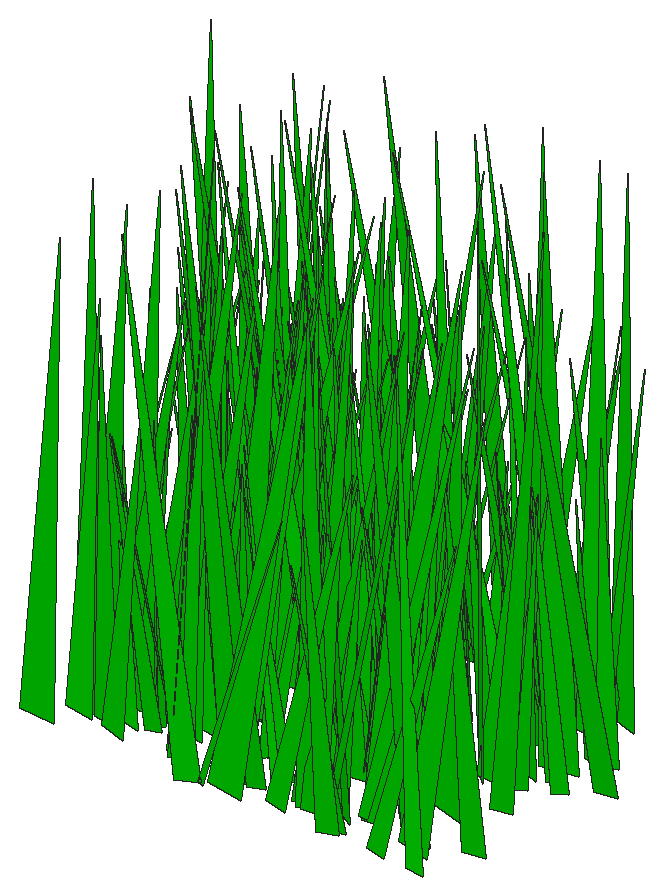
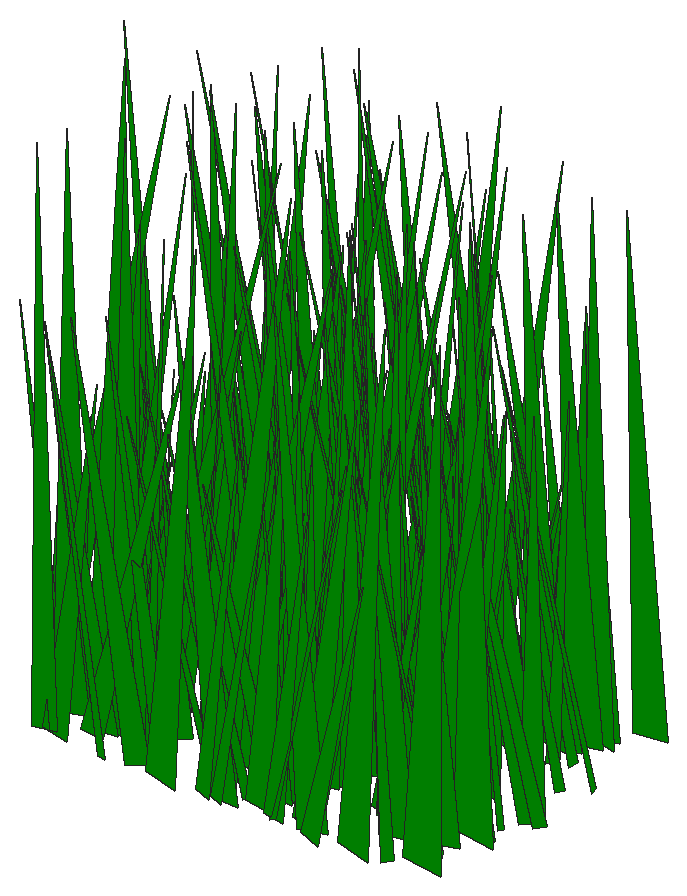
# SketchUp Ruby script. Lengths in inches.
U = 1.inch
M = Sketchup.active_model
def pt(a) = Geom::Point3d.new(a.map { |v| v * U })
def face(e, loops, mat)
  f = e.add_face(loops[0].map { |a| pt(a) })
  loops[1..].each { |l| e.add_face(l.map { |a| pt(a) }).erase! }
  f.material = f.back_material = mat if mat
  f
end
# faces: each face lists its corners as indices into pts; further lists are holes
def faces(e, pts, list, mat = nil) = list.each { |f| face(e, (f[0].is_a?(Array) ? f : [f]).map { |l| l.map { |i| pts[i] } }, mat) }
# xy, xz, yz: faces in a plane at the given z, y or x. An outline is a flat list of corners, or four numbers for a rectangle; further outlines are holes
def ring(l) = l.size == 4 ? [[l[0], l[1]], [l[2], l[1]], [l[2], l[3]], [l[0], l[3]]] : l.each_slice(2).to_a
def flat(e, list, mat, &to3) = list.each { |f| face(e, (f[0].is_a?(Array) ? f : [f]).map { |l| ring(l).map { |u, v| to3.(u, v) } }, mat) }
def xy(e, z, list, mat = nil) = flat(e, list, mat) { |x, y| [x, y, z] }
def xz(e, y, list, mat = nil) = flat(e, list, mat) { |x, z| [x, y, z] }
def yz(e, x, list, mat = nil) = flat(e, list, mat) { |y, z| [x, y, z] }
def lines(e, pts, list) = list.each { |a, b| e.add_line(pt(pts[a]), pt(pts[b])) }
# prism: a flat outline (further loops are holes) pulled along v
def prism(e, loops, v, mat = nil)
  f = face(e, loops, mat); d = Geom::Vector3d.new(v.map { |x| x * U })
  f.pushpull(f.normal.samedirection?(d) ? d.length : -d.length)
end
def box(e, o, s, mat = nil) = prism(e, [[o, [o[0] + s[0], o[1], o[2]], [o[0] + s[0], o[1] + s[1], o[2]], [o[0], o[1] + s[1], o[2]]]], [0, 0, s[2]], mat)
def at(x, y, z, deg = 0) = Geom::Transformation.translation(pt([x, y, z])) * Geom::Transformation.rotation(ORIGIN, Z_AXIS, deg.degrees)
def axes(o, x, y, z) = Geom::Transformation.new([*x, 0, *y, 0, *z, 0, *pt(o).to_a, 1])
def part(name) = M.definitions.add(name)
# library, detail: a bought-in or finely detailed component or shape, given as its bounding box
def library(name, o, s) = part(name).tap { |d| box(d.entities, o, s) }
def detail(e, o, s) = box(e.add_group.entities, o, s)
def put(e, d, t, mat = nil) = e.add_instance(d, t).tap { |i| i.material = mat if mat }
def group(e, t, mat = nil) = e.add_group.tap { |g| g.transformation = t; g.material = mat if mat }.entities
root = M.entities
M.materials.add("[Color G06]").color = [0, 204, 0]
c1 = part("fur_instance\#9")
p = [[0.8125,0,1.79],[0.67,-0.02,1.48],[0,-0.11,0],[0,0.11,0]]
faces(c1.entities,p,[[0,1,2,3]])
put(root,c1,axes([79.69,23.12,4.28],[1.66011,0.80063,2.32778],[5.89187,-0.25245,0.58844],[-0.82253,-0.19243,8.91321]),"[Color G06]")
put(root,c1,axes([79.5,20.96,4.28],[1.87537,-0.4948,0.57966],[-3.50181,-0.26688,-0.86236],[-0.69185,0.00955,5.93611]),"[Color G06]")
put(root,c1,axes([79.8125,25.06,4.28],[0.92833,-0.7609,0.17806],[-5.43768,-0.13039,-0.6811],[-0.46928,0.00566,8.24438]),"[Color G06]")
put(root,c1,axes([80.91,22.99,4.28],[-1.65961,0.74397,0.46911],[5.32789,0.22671,0.80106],[-0.4198,-0.06384,8.31219]),"[Color G06]")
put(root,c1,axes([79.46,16.25,4.28],[0.84063,-0.68793,1.84185],[-5.08275,-0.10859,0.52278],[0.14861,0.17743,7.46121]),"[Color G06]")
put(root,c1,axes([79.29,22.84,4.28],[3.77502,-0.05188,0.90133],[-0.29369,-0.5294,-0.7527],[-0.64486,-0.06259,5.61919]),"[Color G06]")
put(root,c1,axes([79.43,22.34,4.28],[4.54838,0.15375,1.99844],[1.30213,-0.64875,-0.88622],[-1.14373,-0.12715,6.93841]),"[Color G06]")
put(root,c1,axes([80.61,18.76,4.28],[-3.18523,0.26777,1.23981],[1.8153,0.45856,-0.9593],[1.0393,0.01971,5.47532]),"[Color G06]")
put(root,c1,axes([79.5,19.875,4.28],[2.44107,-0.15822,0.6175],[-1.18829,-0.33785,0.54897],[-0.21453,0.07105,3.98557]),"[Color G06]")
put(root,c1,axes([78.86,19.29,4.28],[4.11798,-0.00905,0.35918],[-0.08196,-0.57371,0.43813],[-0.23505,0.04147,6.13978]),"[Color G06]")
put(root,c1,axes([80.37,17.24,4.28],[2.15194,0.68291,2.05903],[4.98687,-0.32442,0.7182],[-1.00627,-0.14733,7.96251]),"[Color G06]")
put(root,c1,axes([79.99,23.87,4.28],[-0.83044,0.54466,1.8968],[4.0338,0.1421,-0.74237],[0.77168,-0.15665,5.92184]),"[Color G06]")
put(root,c1,axes([81.09,21.81,4.28],[-2.89914,0.36743,1.57042],[2.785,0.4085,0.5051],[0.53934,-0.13429,5.8334]),"[Color G06]")
put(root,c1,axes([80.18,17.11,4.28],[2.06618,-0.43483,3.26903],[-3.75525,-0.2906,0.86134],[-0.6372,0.30264,5.52402]),"[Color G06]")
put(root,c1,axes([79.05,21.65,4.28],[2.78739,-0.40955,0.25095],[-2.92397,-0.38217,0.90034],[0.32302,0.07467,5.98435]),"[Color G06]")
put(root,c1,axes([78.74,21.63,4.28],[4.2857,-0.22648,0.18723],[-1.62832,-0.59423,0.68479],[0.04588,0.06593,6.8155]),"[Color G06]")
put(root,c1,axes([80.87,21.13,4.28],[0.30807,-0.52519,1.37822],[-3.85703,-0.05476,-0.47116],[-0.39833,0.12403,5.62812]),"[Color G06]")
put(root,c1,axes([81.37,21.29,4.28],[-2.88507,0.05319,0.98148],[0.52408,0.39979,0.95244],[0.54961,-0.10202,4.2439]),"[Color G06]")
put(root,c1,axes([80.93,22.57,4.28],[-2.8721,0.2607,2.58131],[2.25164,0.42956,0.6126],[1.18669,-0.18408,5.08509]),"[Color G06]")
put(root,c1,axes([80.65,25.42,4.28],[2.59498,-0.18041,1.97945],[-1.60015,-0.3785,0.72288],[-0.93141,0.14761,4.27299]),"[Color G06]")
put(root,c1,axes([80.1,23.22,4.28],[3.23235,0.00995,0.84721],[0.18253,-0.44833,-0.95061],[-0.54139,-0.09173,4.73774]),"[Color G06]")
put(root,c1,axes([80.84,22.36,4.28],[3.4788,0.05812,2.24825],[0.64999,-0.51979,-0.70299],[-1.41918,-0.0956,5.1891]),"[Color G06]")
put(root,c1,axes([80.47,17.64,4.28],[0.16871,-0.7141,2.41207],[-5.34596,-0.00136,0.78909],[0.50038,0.22627,7.61715]),"[Color G06]")
put(root,c1,axes([79.73,24.36,4.28],[3.97397,0.03639,0.40781],[0.21667,-0.54926,0.91315],[-0.30918,0.08275,5.88172]),"[Color G06]")
put(root,c1,axes([81.11,17.11,4.28],[-1.43177,-0.51905,1.38849],[-3.78293,0.21402,0.47736],[0.63854,0.1041,5.94141]),"[Color G06]")
put(root,c1,axes([81.66,25.5625,4.28],[-2.49264,-0.58211,3.3509],[-4.71114,0.34234,-0.99648],[0.5082,0.31838,7.19804]),"[Color G06]")
put(root,c1,axes([81.18,21.12,4.28],[-1.98811,-0.36527,1.43701],[-2.64413,0.29921,0.56523],[0.89129,0.07287,4.88223]),"[Color G06]")
put(root,c1,axes([80.39,19.99,4.28],[1.88128,0.50127,1.10467],[3.6688,-0.25399,-0.71661],[0.09149,-0.12219,6.02138]),"[Color G06]")
put(root,c1,axes([82.73,22.41,4.28],[-3.96799,-0.55484,1.07641],[-4.039,0.55053,-0.65975],[0.19187,0.11471,8.37251]),"[Color G06]")
put(root,c1,axes([80.95,19.18,4.28],[2.7584,0.16784,1.74145],[1.45516,-0.39514,-0.77369],[-0.83001,-0.13496,4.43098]),"[Color G06]")
put(root,c1,axes([81.68,17.37,4.28],[-1.79244,0.34364,0.09023],[2.42373,0.24758,-0.76576],[0.44943,0.03532,4.48948]),"[Color G06]")
put(root,c1,axes([80.09,18.58,4.28],[4.14622,-0.10146,0.80041],[-0.78731,-0.57782,0.69621],[-0.44309,0.07732,6.25287]),"[Color G06]")
put(root,c1,axes([81.26,18.12,4.28],[1.25653,0.77587,0.32967],[5.5557,-0.17681,0.50029],[-0.37526,-0.01966,8.51051]),"[Color G06]")
put(root,c1,axes([82.45,23.49,4.28],[-2.60406,0.26968,1.00772],[2.03612,0.35729,0.7692],[0.22103,-0.1142,4.78643]),"[Color G06]")
put(root,c1,axes([82.35,17.52,4.28],[-1.28233,-0.37257,0.8641],[-2.72776,0.16854,-0.69447],[-0.17974,0.10035,4.37457]),"[Color G06]")
put(root,c1,axes([81.25,24.31,4.28],[1.6658,-0.65409,2.38531],[-4.9522,-0.22726,0.56649],[-0.15747,0.22769,7.41785]),"[Color G06]")
put(root,c1,axes([81.02,22.03,4.28],[2.14567,-0.34921,1.40037],[-2.67112,-0.28745,0.90769],[-0.11976,0.1548,4.84443]),"[Color G06]")
put(root,c1,axes([80.61,18.15,4.28],[2.90085,-0.50873,0.70298],[-3.67786,-0.39967,0.67542],[0.06417,0.09052,6.93331]),"[Color G06]")
put(root,c1,axes([81.92,23.74,4.28],[3.83414,-0.45659,2.9579],[-3.37058,-0.58797,-0.66671],[-1.81029,0.1277,7.5061]),"[Color G06]")
put(root,c1,axes([81.78,20.38,4.28],[-2.1759,0.53004,2.48183],[3.95463,0.34398,-0.6944],[1.25155,-0.1654,6.50898]),"[Color G06]")
put(root,c1,axes([81.875,19.92,4.28],[3.59238,0.2328,2.12613],[1.68174,-0.53673,0.40383],[-1.40805,-0.0471,5.90675]),"[Color G06]")
put(root,c1,axes([81.11,23.89,4.28],[5.55783,0.14859,2.34897],[1.26478,-0.79531,-0.90529],[-1.41631,-0.12712,8.40929]),"[Color G06]")
put(root,c1,axes([82.92,25.74,4.28],[-1.05256,-0.36083,0.66501],[-2.5884,0.13139,-0.9615],[-0.44028,0.09016,4.06285]),"[Color G06]")
put(root,c1,axes([83.08,17.53,4.28],[-3.04542,-0.12878,0.21028],[-0.88398,0.4189,0.87378],[0.30218,-0.0725,4.67535]),"[Color G06]")
put(root,c1,axes([81.58,16.77,4.28],[-0.58854,-0.46279,1.67623],[-3.39274,0.11481,0.98036],[0.87278,0.13421,4.9413]),"[Color G06]")
put(root,c1,axes([81.09,23.79,4.28],[5.54522,0.11295,2.02169],[0.92552,-0.79156,-0.5901],[-1.27645,-0.08324,8.35488]),"[Color G06]")
put(root,c1,axes([82.39,17.85,4.28],[-2.61219,-0.15207,1.92785],[-1.37634,0.38366,-0.68921],[0.97919,0.13358,4.17417]),"[Color G06]")
put(root,c1,axes([82.15,18.91,4.28],[2.63972,0.31328,2.14311],[2.53839,-0.38129,-0.58123],[-0.81232,-0.17347,5.14793]),"[Color G06]")
put(root,c1,axes([83.83,24.25,4.28],[-3.35141,-0.32704,0.66967],[-2.38616,0.46258,-0.72411],[0.08509,0.09126,6.07051]),"[Color G06]")
put(root,c1,axes([81.03,23.02,4.28],[5.13435,-0.0033,0.87473],[0.02683,-0.71794,-0.66265],[-0.58513,-0.06185,7.64507]),"[Color G06]")
put(root,c1,axes([82.16,22.1,4.28],[3.34124,0.17837,1.87886],[1.48232,-0.4833,-0.61772],[-1.00955,-0.1193,5.31135]),"[Color G06]")
put(root,c1,axes([83.42,25.22,4.28],[-1.08926,-0.58418,1.11674],[-4.24517,0.14171,-0.73383],[-0.29541,0.11767,6.42769]),"[Color G06]")
put(root,c1,axes([82.18,18.59,4.28],[5.61497,0.11011,2.71942],[0.6333,-0.82141,0.89966],[-1.87966,0.05216,8.42666]),"[Color G06]")
put(root,c1,axes([83.37,21.68,4.28],[-2.92894,0.18384,1.54457],[1.49028,0.41852,0.59019],[0.76497,-0.11145,4.76412]),"[Color G06]")
put(root,c1,axes([82.19,23.43,4.28],[3.59135,-0.1809,0.95601],[-1.23494,-0.50779,-0.67547],[-0.75306,-0.03001,5.66688]),"[Color G06]")
put(root,c1,axes([83.53,18.36,4.28],[-1.79738,0.36474,0.18272],[2.59187,0.25076,-0.55029],[0.37245,0.01514,4.71124]),"[Color G06]")
put(root,c1,axes([84.28,25.52,4.28],[-3.44278,-0.19488,0.37051],[-1.3531,0.47802,0.79821],[0.42864,-0.05629,5.49561]),"[Color G06]")
put(root,c1,axes([83.12,17.94,4.28],[-1.33051,0.65402,1.71855],[4.73734,0.20903,-0.9458],[0.93666,-0.12821,7.22473]),"[Color G06]")
put(root,c1,axes([83.67,21.57,4.28],[-3.7587,0.44327,3.41119],[3.64212,0.55767,0.63959],[1.4315,-0.25497,7.32946]),"[Color G06]")
put(root,c1,axes([82.42,19.19,4.28],[2.84863,0.50988,1.46683],[3.78266,-0.39041,-0.81971],[-0.15668,-0.15525,6.87889]),"[Color G06]")
put(root,c1,axes([84.38,19.74,4.28],[-5.10731,0.29208,1.74483],[2.02134,0.73046,-0.83029],[1.29011,0.0118,8.20836]),"[Color G06]")
put(root,c1,axes([82.98,21.77,4.28],[2.77048,-0.07926,0.83529],[-0.45684,-0.38885,-0.85393],[-0.65324,-0.06422,4.13978]),"[Color G06]")
put(root,c1,axes([84.73,15.98,4.28],[-4.04853,0.48437,1.71639],[3.61711,0.56576,0.71717],[0.54843,-0.1558,7.94035]),"[Color G06]")
put(root,c1,axes([83.12,20.18,4.28],[4.69266,0.00046,2.39144],[0.19454,-0.6864,-0.83759],[-1.58822,-0.08272,6.96333]),"[Color G06]")
put(root,c1,axes([84.53,18.45,4.28],[-4.20784,-0.54749,1.06663],[-3.89161,0.59499,0.79008],[0.883,0.0133,8.56502]),"[Color G06]")
put(root,c1,axes([83.2,21.58,4.28],[1.20975,0.55134,1.81595],[4.13607,-0.16299,-0.47022],[-0.04089,-0.17493,6.16173]),"[Color G06]")
put(root,c1,axes([83.85,23.14,4.28],[1.48292,0.70244,2.85752],[5.32505,-0.23322,0.41283],[-0.82118,-0.24383,7.8373]),"[Color G06]")
put(root,c1,axes([84.3,25.47,4.28],[-1.61808,0.35016,1.36109],[2.66901,0.21785,0.64927],[0.10628,-0.13992,4.41722]),"[Color G06]")
put(root,c1,axes([83.1,25.39,4.28],[2.58622,-0.57699,2.32565],[-4.39907,-0.36074,0.64604],[-0.43676,0.21681,7.26413]),"[Color G06]")
put(root,c1,axes([82.375,18.07,4.28],[3.9356,-0.64285,1.08446],[-4.66141,-0.54786,0.48052],[-0.22419,0.10616,9.04657]),"[Color G06]")
put(root,c1,axes([83.93,24.48,4.28],[1.63087,0.42435,1.56238],[3.10237,-0.25073,0.58922],[-0.85362,-0.10051,5.12639]),"[Color G06]")
put(root,c1,axes([83.65,16.74,4.28],[2.7912,0.29184,1.36812],[2.05108,-0.40891,0.67289],[-1.00549,-0.024,5.17047]),"[Color G06]")
put(root,c1,axes([82.94,19.77,4.28],[3.60408,0.24247,0.53661],[1.68649,-0.50293,0.8041],[-0.55516,0.04628,5.92641]),"[Color G06]")
put(root,c1,axes([85.31,21.05,4.28],[-3.32652,-0.53113,0.78703],[-3.84506,0.45979,-0.65782],[0.01178,0.09569,7.52935]),"[Color G06]")
put(root,c1,axes([84.92,22.2,4.28],[-3.6077,-0.0724,1.02155],[-0.62929,0.50315,-0.86794],[0.58373,0.09495,5.37794]),"[Color G06]")
put(root,c1,axes([84.26,23.33,4.28],[-3.87405,-0.51095,2.30567],[-3.70724,0.57277,0.667],[1.43609,0.10024,7.94168]),"[Color G06]")
put(root,c1,axes([84.71,22.05,4.28],[-2.95724,0.47679,0.3907],[3.37782,0.41331,-0.83187],[0.59139,0.0235,6.70504]),"[Color G06]")
put(root,c1,axes([83.77,16.87,4.28],[-0.63586,0.55558,1.45196],[4.05107,0.10641,-0.71449],[0.6376,-0.12203,5.98757]),"[Color G06]")
put(root,c1,axes([83.89,24.43,4.28],[2.5775,0.09656,1.50917],[0.88481,-0.37372,-0.62873],[-0.8463,-0.09665,3.93899]),"[Color G06]")
put(root,c1,axes([84.03,19.33,4.28],[2.46724,0.25141,1.12453],[1.71569,-0.35967,0.82874],[-0.93434,0.00342,4.49125]),"[Color G06]")
put(root,c1,axes([85.95,20.1,4.28],[-5.42016,-0.36928,1.14945],[-2.71155,0.75675,-0.63262],[0.50199,0.10043,8.9938]),"[Color G06]")
put(root,c1,axes([85.1,17.625,4.28],[-2.38817,-0.74727,2.22841],[-5.56124,0.32549,-0.77439],[0.11624,0.21951,8.73434]),"[Color G06]")
put(root,c1,axes([83.79,22.21,4.28],[-0.42686,0.46146,2.9038],[3.77293,0.10025,-0.59115],[0.70074,-0.25864,4.95175]),"[Color G06]")
put(root,c1,axes([82.37,21.99,4.28],[4.94318,0.30244,0.62335],[2.20504,-0.68389,-0.94278],[-0.12511,-0.104,8.01251]),"[Color G06]")
put(root,c1,axes([84.27,24.5,4.28],[-1.62976,-0.49759,1.66629],[-3.64862,0.24867,0.55899],[0.81475,0.11825,5.83639]),"[Color G06]")
put(root,c1,axes([83.98,20.03,4.28],[2.2929,-0.23561,1.3779],[-1.85184,-0.32456,0.50833],[-0.52481,0.11585,4.22636]),"[Color G06]")
put(root,c1,axes([84.05,22.45,4.28],[3.98863,0.32722,1.7603],[2.25756,-0.57993,0.95726],[-1.3405,-0.00304,6.84986]),"[Color G06]")
put(root,c1,axes([84.93,25.25,4.28],[-0.03064,-0.53308,1.7802],[-3.985,-0.01215,-0.5712],[-0.39079,0.1657,5.68509]),"[Color G06]")
put(root,c1,axes([85.55,21.73,4.28],[-0.70137,0.79473,0.36072],[5.668,0.09327,1.01148],[-0.64302,-0.04471,8.52238]),"[Color G06]")
put(root,c1,axes([83.28,21.58,4.28],[4.04149,0.19855,0.15121],[1.42519,-0.55889,-0.78533],[0.07995,-0.07378,6.35587]),"[Color G06]")
put(root,c1,axes([84.11,18.82,4.28],[1.87067,-0.78026,1.23723],[-5.65466,-0.255,0.6239],[0.13796,0.12784,8.79567]),"[Color G06]")
put(root,c1,axes([84.39,21.38,4.28],[2.44326,0.45611,1.95979],[3.49775,-0.34096,-0.62479],[-0.42884,-0.18236,6.06979]),"[Color G06]")
put(root,c1,axes([84.53,24.65,4.28],[2.87126,-0.17062,1.04083],[-1.18824,-0.41199,-0.43638],[-0.75513,-0.00047,4.64426]),"[Color G06]")
put(root,c1,axes([84.93,20.6,4.28],[3.42781,-0.2245,1.82832],[-1.55616,-0.50729,-0.63855],[-1.29106,0.01539,5.62392]),"[Color G06]")
put(root,c1,axes([85.67,19.84,4.28],[-4.16333,-0.05682,1.93724],[-0.253,0.60482,0.82312],[1.33495,-0.06257,6.19771]),"[Color G06]")
put(root,c1,axes([87,23.78,4.28],[-3.88284,0.58889,0.3395],[4.22384,0.53782,0.74185],[-0.21251,-0.07011,8.54191]),"[Color G06]")
put(root,c1,axes([86.39,19.93,4.28],[-4.95009,-0.52248,1.03667],[-3.68816,0.6968,1.00405],[0.95778,-0.01713,9.22418]),"[Color G06]")
put(root,c1,axes([84.88,23.125,4.28],[3.14975,0.47083,3.24548],[3.90167,-0.44963,-0.96498],[-0.94498,-0.28711,6.83342]),"[Color G06]")
put(root,c1,axes([86.02,25.65,4.28],[-2.71853,0.14993,1.15323],[1.24468,0.37318,0.98075],[0.44962,-0.12657,4.25778]),"[Color G06]")
put(root,c1,axes([84.8125,21.02,4.28],[0.51696,0.48605,1.36335],[3.58432,-0.05631,-0.72957],[0.36624,-0.13493,5.21568]),"[Color G06]")
put(root,c1,axes([86.38,16.82,4.28],[-3.7856,-0.42403,1.87518],[-3.23668,0.52776,-0.88631],[0.58726,0.17533,7.20284]),"[Color G06]")
put(root,c1,axes([87.32,18.74,4.28],[-4.90014,0.48636,0.13008],[3.47735,0.68253,-0.54937],[0.28395,0.03474,8.97258]),"[Color G06]")
put(root,c1,axes([86.65,24.71,4.28],[-3.2921,-0.70067,1.74882],[-5.14871,0.45849,-0.54815],[0.32752,0.16478,8.9613]),"[Color G06]")
put(root,c1,axes([85.36,23.17,4.28],[1.44736,-0.39047,2.05591],[-3.09984,-0.20388,0.42638],[-0.35252,0.18963,4.69175]),"[Color G06]")
put(root,c1,axes([85.32,23.03,4.28],[-0.87579,0.41999,1.30902],[3.02509,0.14661,-0.88288],[0.8291,-0.0913,4.60404]),"[Color G06]")
put(root,c1,axes([85.9,16.98,4.28],[1.06266,0.41431,1.18108],[3.00606,-0.16448,0.58639],[-0.6449,-0.08396,4.6795]),"[Color G06]")
put(root,c1,axes([83.86,19.74,4.28],[4.18548,-0.55342,0.19963],[-3.96114,-0.57996,0.81654],[0.27953,0.06806,8.58185]),"[Color G06]")
put(root,c1,axes([84.86,24.76,4.28],[1.25588,0.42099,0.01724],[2.96201,-0.17148,-0.95261],[0.58415,-0.03559,4.79327]),"[Color G06]")
put(root,c1,axes([86.48,25.63,4.28],[-2.79493,-0.29953,1.50457],[-2.29381,0.39655,-0.44948],[0.6047,0.11981,5.24912]),"[Color G06]")
put(root,c1,axes([86.78,23.3,4.28],[-2.12689,-0.23326,0.5564],[-1.71354,0.29049,-0.64214],[0.02081,0.07922,3.99282]),"[Color G06]")
put(root,c1,axes([87.77,20.63,4.28],[-5.51697,0.4026,1.25408],[2.96376,0.76935,0.75147],[0.50577,-0.11676,9.27596]),"[Color G06]")
put(root,c1,axes([84.97,17.77,4.28],[4.63675,-0.22525,1.71691],[-1.73208,-0.65859,0.52312],[-0.9638,0.0999,7.31979]),"[Color G06]")
put(root,c1,axes([86.79,17.57,4.28],[-1.67886,0.32432,0.38148],[2.33804,0.23088,0.43604],[-0.08887,-0.05262,4.26481]),"[Color G06]")
put(root,c1,axes([85.52,18.17,4.28],[3.52781,-0.14791,1.32934],[-0.98718,-0.50685,-0.62641],[-0.9704,-0.0221,5.46998]),"[Color G06]")
put(root,c1,axes([86.83,17.1,4.28],[-3.22267,0.13531,1.09509],[0.92789,0.46073,-0.43986],[0.78575,0.01087,5.01083]),"[Color G06]")
put(root,c1,axes([85.82,22.64,4.28],[3.20574,0.18951,1.89514],[1.57129,-0.46462,-0.59995],[-0.99291,-0.1234,5.16928]),"[Color G06]")
put(root,c1,axes([84.97,20.27,4.28],[4.20872,0.15744,0.27612],[1.10328,-0.58453,0.722],[-0.30262,0.05849,6.4725]),"[Color G06]")
put(root,c1,axes([85.07,16.09,4.28],[3.29273,-0.04593,0.05053],[-0.33083,-0.45451,0.69821],[0.0132,0.06529,4.89625]),"[Color G06]")
put(root,c1,axes([86.28,20.09,4.28],[2.46649,0.73853,1.11728],[5.26779,-0.3553,1.00288],[-0.92676,-0.05405,8.67406]),"[Color G06]")
put(root,c1,axes([87.14,21.04,4.28],[-0.4718,-0.69691,0.31053],[-4.98676,0.06326,-0.61498],[-0.39054,0.03414,7.47741]),"[Color G06]")
put(root,c1,axes([85.6875,18.27,4.28],[3.21881,-0.20248,0.90509],[-1.52144,-0.44956,0.53315],[-0.40037,0.08055,5.25057]),"[Color G06]")
put(root,c1,axes([85.18,22.07,4.28],[3.80931,0.44972,0.68766],[3.25673,-0.52813,-0.62206],[-0.07986,-0.0858,7.43369]),"[Color G06]")
put(root,c1,axes([85.44,25.1,4.28],[3.373,0.23491,0.46266],[1.71279,-0.4621,-0.94011],[0.00894,-0.09775,5.55599]),"[Color G06]")
put(root,c1,axes([87.54,23.06,4.28],[-0.65547,-0.46448,1.16801],[-3.38418,0.0717,-0.96678],[-0.50316,0.12284,4.98083]),"[Color G06]")
put(root,c1,axes([85.85,25.59,4.28],[3.1327,-0.56366,0.15371],[-4.03031,-0.43674,-0.49759],[-0.32607,-0.01713,7.62703]),"[Color G06]")
put(root,c1,axes([87.89,19.51,4.28],[-2.2816,0.39241,0.68252],[2.84951,0.31137,0.713],[-0.0884,-0.09126,5.3674]),"[Color G06]")
put(root,c1,axes([85.82,16.17,4.28],[2.32743,0.73838,0.05758],[5.2832,-0.32341,-0.60753],[0.35667,-0.02771,8.62327]),"[Color G06]")
put(root,c1,axes([86.8,22.79,4.28],[1.91769,0.46471,0.13215],[3.29065,-0.26614,0.84604],[-0.53439,0.02881,5.68394]),"[Color G06]")
put(root,c1,axes([87.76,25.74,4.28],[2.31683,0.58899,3.72552],[4.5987,-0.3945,0.77637],[-1.70461,-0.26376,7.15807]),"[Color G06]")
put(root,c1,axes([86.51,24.79,4.28],[3.1907,-0.30441,0.90845],[-2.1553,-0.45288,-0.52354],[-0.69982,0.00685,5.7543]),"[Color G06]")
put(root,c1,axes([85.77,16.85,4.28],[5.14575,-0.3356,1.57178],[-2.51936,-0.72187,0.71798],[-0.74222,0.12362,8.45987]),"[Color G06]")
put(root,c1,axes([86.12,22.44,4.28],[2.1675,-0.53809,0.02462],[-3.84702,-0.30112,0.53044],[0.3014,0.02623,6.59346]),"[Color G06]")
put(root,c1,axes([86.39,20.94,4.28],[2.05528,-0.63608,0.92944],[-4.59875,-0.27926,0.76104],[0.21369,0.10805,7.43876]),"[Color G06]")
put(root,c1,axes([86.16,24.91,4.28],[4.09837,-0.05278,0.47946],[-0.41506,-0.56863,0.73491],[-0.2718,0.07257,6.10731]),"[Color G06]")
put(root,c1,axes([87.15,22.15,4.28],[2.52289,0.33235,0.86172],[2.37296,-0.35998,0.43004],[-0.61798,-0.02546,5.16928]),"[Color G06]")
put(root,c1,axes([88.04,18.85,4.28],[1.42557,0.50992,2.73226],[3.95235,-0.24093,0.55895],[-1.04538,-0.21554,5.83922]),"[Color G06]")
put(root,c1,axes([87.56,17.97,4.28],[-0.32043,-0.37537,0.61921],[-2.70497,0.05065,0.40029],[0.31777,0.05262,4.03179]),"[Color G06]")
put(root,c1,axes([87.32,19.6875,4.28],[-3.07301,0.57405,3.34534],[4.29713,0.49409,-0.92227],[1.86865,-0.19216,7.62228]),"[Color G06]")
put(root,c1,axes([86.45,22.87,4.28],[4.73035,0.461,1.85384],[3.47171,-0.65998,-0.93486],[-0.64421,-0.17163,8.57451]),"[Color G06]")
put(root,c1,axes([88.625,19.6,4.28],[-4.10955,0.10491,1.89038],[0.95934,0.58769,0.91195],[1.116,-0.11887,6.17715]),"[Color G06]")
put(root,c1,axes([86.64,25,4.28],[3.53184,-0.07964,0.1681],[-0.57937,-0.49028,0.50745],[-0.0563,0.04925,5.32304]),"[Color G06]")
put(root,c1,axes([88.55,23.14,4.28],[-4.35819,-0.05811,2.26646],[-0.56435,0.63929,-0.54125],[1.46792,0.07326,6.52092]),"[Color G06]")
put(root,c1,axes([88.07,17.05,4.28],[5.13413,-0.21655,3.69857],[-1.8426,-0.78147,0.45728],[-2.26727,0.14472,8.00362]),"[Color G06]")
put(root,c1,axes([86.88,18.66,4.28],[4.26032,0.38989,0.36075],[2.77377,-0.5943,0.61439],[-0.42695,0.02957,7.59136]),"[Color G06]")
put(root,c1,axes([87.74,21.78,4.28],[1.72097,0.32647,1.0854],[2.44593,-0.23688,-0.47816],[-0.1618,-0.10834,4.31638]),"[Color G06]")
put(root,c1,axes([87.95,20.18,4.28],[1.0671,-0.67021,3.70909],[-5.40901,-0.1348,0.67803],[-0.03965,0.35175,7.32691]),"[Color G06]")
put(root,c1,axes([89.18,23.09,4.28],[-3.38666,-0.36972,0.494],[-2.59796,0.47304,0.88587],[0.62424,-0.03713,6.36694]),"[Color G06]")
put(root,c1,axes([88.28,16.86,4.28],[1.74083,-0.72372,0.98893],[-5.18663,-0.25149,-0.7478],[-0.68736,0.06476,8.14726]),"[Color G06]")
put(root,c1,axes([87.76,21.8,4.28],[1.38063,0.45134,1.21851],[3.33533,-0.18185,-0.70365],[0.12751,-0.13007,5.21185]),"[Color G06]")
put(root,c1,axes([88.92,21.97,4.28],[-4.69419,0.51555,2.55516],[3.71454,0.69108,-0.77454],[1.67153,-0.0879,8.8969]),"[Color G06]")
put(root,c1,axes([87.59,16.94,4.28],[4.43568,0.21649,1.28625],[1.48529,-0.62953,0.73067],[-0.97208,0.02598,6.98569]),"[Color G06]")
put(root,c1,axes([88.24,21.37,4.28],[0.56782,-0.35012,1.24979],[-2.64333,-0.06932,0.4517],[0.12677,0.12272,3.82069]),"[Color G06]")
put(root,c1,axes([87.37,16.38,4.28],[2.97188,-0.37393,0.4675],[-2.69399,-0.40652,0.90191],[0.17591,0.09155,5.91416]),"[Color G06]")
put(root,c1,axes([88.95,24.67,4.28],[4.51624,-0.12207,3.27441],[-0.71853,-0.69962,-0.78254],[-2.24721,-0.02163,6.83081]),"[Color G06]")
put(root,c1,axes([90.99,21.93,4.28],[-5.78696,0.34164,0.04351],[2.44421,0.80567,-0.55308],[0.17104,0.04594,9.37594]),"[Color G06]")
put(root,c1,axes([89.61,16.29,4.28],[-1.86922,-0.27751,0.40706],[-2.00854,0.25768,-0.42237],[-0.02155,0.05465,4.05871]),"[Color G06]")
put(root,c1,axes([89.28,16.96,4.28],[3.83621,0.16577,3.62261],[1.5495,-0.61613,-0.42646],[-2.21073,-0.14419,5.98732]),"[Color G06]")
put(root,c1,axes([88,19.32,4.28],[4.90041,0.09712,1.74017],[0.56831,-0.69947,0.90967],[-1.23198,0.06365,7.34148]),"[Color G06]")
put(root,c1,axes([88.62,23.6875,4.28],[-1.06421,0.34027,0.9736],[2.39387,0.16732,-0.87256],[0.805,-0.04773,3.88186]),"[Color G06]")
put(root,c1,axes([88.39,16.72,4.28],[3.82743,0.59771,1.8736],[4.32187,-0.55373,0.57132],[-1.12495,-0.09376,8.56948]),"[Color G06]")
put(root,c1,axes([90.6,24.95,4.28],[-3.69965,0.3937,0.19743],[2.82156,0.51266,0.66613],[-0.16597,-0.06055,6.92362]),"[Color G06]")
put(root,c1,axes([89.35,16.09,4.28],[0.44074,-0.48379,0.37331],[-3.44186,-0.06573,-0.70818],[-0.50244,0.02589,5.1787]),"[Color G06]")
put(root,c1,axes([90.42,24.26,4.28],[-5.42402,0.36649,1.27411],[2.56942,0.76535,-0.85586],[1.01589,0.02098,8.96735]),"[Color G06]")
put(root,c1,axes([88.125,25.15,4.28],[3.78273,-0.30943,0.65818],[-2.19362,-0.53094,-0.51233],[-0.553,-0.01046,6.53445]),"[Color G06]")
put(root,c1,axes([88.88,17.14,4.28],[0.32871,-0.39632,1.18726],[-2.93181,-0.03116,0.61836],[0.33624,0.11576,4.23109]),"[Color G06]")
put(root,c1,axes([89.72,18.09,4.28],[-2.49154,-0.16723,1.6311],[-1.39159,0.36374,-0.46417],[0.83233,0.10754,4.10656]),"[Color G06]")
put(root,c1,axes([90.66,23.2,4.28],[-2.53013,-0.41362,0.90276],[-3.02569,0.34224,-0.92887],[-0.0915,0.12018,5.75239]),"[Color G06]")
put(root,c1,axes([89.83,19.42,4.28],[-2.8498,0.27125,1.38855],[1.90915,0.4173,-0.61216],[1.00105,-0.02367,5.12039]),"[Color G06]")
put(root,c1,axes([89.11,24.57,4.28],[-1.70895,-0.37741,2.45877],[-2.88607,0.29293,0.68439],[1.30464,0.15365,4.73471]),"[Color G06]")
put(root,c1,axes([89.81,24.48,4.28],[-2.60805,0.73404,2.33271],[5.3795,0.38983,-0.65664],[1.09831,-0.16633,8.75547]),"[Color G06]")
put(root,c1,axes([90.52,18.04,4.28],[-1.4419,-0.38439,0.85097],[-2.80954,0.19111,-0.71716],[-0.17151,0.10104,4.59386]),"[Color G06]")
put(root,c1,axes([88.7,25.49,4.28],[2.63451,-0.46803,1.05964],[-3.42985,-0.35703,0.93259],[0.06452,0.13139,6.30856]),"[Color G06]")
put(root,c1,axes([89.58,19.37,4.28],[2.80431,-0.11718,1.63108],[-1.04313,-0.4061,0.65457],[-0.89948,0.10563,4.32614]),"[Color G06]")
put(root,c1,axes([88.8,18.98,4.28],[2.46207,0.74351,0.4965],[5.33839,-0.34047,-0.56281],[0.20344,-0.06402,8.75945]),"[Color G06]")
put(root,c1,axes([89.63,22.97,4.28],[0.86197,-0.44373,0.19576],[-3.17522,-0.11827,0.43515],[0.24713,0.02818,4.90806]),"[Color G06]")
put(root,c1,axes([90.94,23.27,4.28],[-2.70464,-0.01988,0.5901],[-0.05784,0.3732,0.85215],[0.41578,-0.0774,3.95718]),"[Color G06]")
put(root,c1,axes([90.64,21.29,4.28],[-0.92937,-0.39325,1.52289],[-2.99856,0.12229,-0.46002],[0.00814,0.14842,4.41397]),"[Color G06]")
put(root,c1,axes([88.98,16.54,4.28],[5.20895,0.23431,0.80155],[1.61451,-0.72729,0.98567],[-0.71013,0.06515,8.12057]),"[Color G06]")
put(root,c1,axes([90.57,23.79,4.28],[-1.62051,-0.69532,0.2363],[-4.9458,0.22695,0.95088],[0.65385,-0.00662,7.77821]),"[Color G06]")
put(root,c1,axes([90.06,17.26,4.28],[2.45987,0.66315,0.73884],[4.74978,-0.34781,0.53792],[-0.54765,-0.03793,7.98406]),"[Color G06]")
put(root,c1,axes([89.9,22.54,4.28],[0.94563,-0.34219,1.53324],[-2.63865,-0.10163,1.02974],[0.33409,0.1659,3.79316]),"[Color G06]")
put(root,c1,axes([90.63,20.9375,4.28],[5.12601,0.12007,3.66843],[1.17973,-0.78142,-0.74407],[-2.31825,-0.13215,7.73282]),"[Color G06]")
put(root,c1,axes([89.66,25.73,4.28],[4.10476,-0.08624,1.06174],[-0.54944,-0.579,-0.65755],[-0.76501,-0.04687,6.16916]),"[Color G06]")
put(root,c1,axes([91.35,25.51,4.28],[-1.07717,-0.47865,1.18041],[-3.51621,0.13943,-0.67275],[-0.20508,0.1235,5.33454]),"[Color G06]")
put(root,c1,axes([91.42,17.23,4.28],[-2.82568,-0.6474,0.82603],[-4.64572,0.39891,0.41654],[0.52627,0.04544,8.11224]),"[Color G06]")
put(root,c1,axes([91.13,21.7,4.28],[2.76854,0.08716,2.35904],[0.35131,-0.44135,0.95223],[-1.6609,0.05193,4.13366]),"[Color G06]")
put(root,c1,axes([91.5,22.95,4.28],[0.06705,-0.39986,1.1314],[-2.91226,-0.02884,-0.78536],[-0.56072,0.10197,4.21432]),"[Color G06]")
put(root,c1,axes([90.39,24.68,4.28],[1.46364,0.555,0.13792],[3.97359,-0.20281,-0.44037],[0.24483,-0.02623,6.32264]),"[Color G06]")
put(root,c1,axes([91.08,18.9,4.28],[-2.4492,-0.62412,2.70681],[-4.59456,0.3883,0.99873],[1.48396,0.17217,7.55967]),"[Color G06]")
put(root,c1,axes([91.52,21.83,4.28],[-3.31101,-0.36635,2.42237],[-2.69606,0.50461,0.53508],[1.50341,0.09809,6.29439]),"[Color G06]")
put(root,c1,axes([89.76,17.3,4.28],[5.13162,-0.29867,0.86361],[-2.19478,-0.71308,0.80172],[-0.32303,0.10029,8.27206]),"[Color G06]")
put(root,c1,axes([91.64,24.4375,4.28],[-2.60388,0.73489,1.92214],[5.30787,0.38621,-0.90084],[1.11985,-0.12182,8.73916]),"[Color G06]")
put(root,c1,axes([90.88,20.97,4.28],[1.8641,-0.45707,1.01985],[-3.34787,-0.25561,0.50922],[-0.03497,0.10624,5.61264]),"[Color G06]")
put(root,c1,axes([91.15,21.54,4.28],[0.7612,0.40267,1.14411],[2.97269,-0.09117,-0.73173],[0.29624,-0.11979,4.40287]),"[Color G06]")
put(root,c1,axes([92.32,21.95,4.28],[-0.10562,0.40942,0.42188],[2.89729,0.00702,0.83806],[-0.553,-0.04144,4.31027]),"[Color G06]")
put(root,c1,axes([92,22.51,4.28],[1.14243,-0.82216,2.4651],[-6.08453,-0.17841,-0.53647],[-0.67864,0.21552,8.95971]),"[Color G06]")
put(root,c1,axes([91.72,25.48,4.28],[-3.5237,-0.56894,3.03761],[-4.1825,0.54598,0.90946],[1.81213,0.15385,8.00575]),"[Color G06]")
put(root,c1,axes([91.86,21.05,4.28],[1.90446,0.36039,0.47784],[2.51779,-0.26892,0.88447],[-0.66518,0.01392,4.71591]),"[Color G06]")
put(root,c1,axes([92.43,15.91,4.28],[-4.53056,0.28903,2.32684],[2.02421,0.66753,-0.72129],[1.61943,-0.02578,7.41122]),"[Color G06]")
put(root,c1,axes([93.78,22.26,4.28],[-4.53351,-0.58052,1.12772],[-4.22669,0.62828,-0.80213],[0.18793,0.12643,9.16401]),"[Color G06]")
put(root,c1,axes([92.42,23.38,4.28],[-1.47324,-0.3352,0.51987],[-2.38218,0.21048,0.51041],[0.47381,0.01598,4.1827]),"[Color G06]")
put(root,c1,axes([92.8125,21.54,4.28],[1.15842,-0.3433,2.14168],[-2.65184,-0.20874,-0.6396],[-1.04015,0.14984,4.01581]),"[Color G06]")
put(root,c1,axes([91,16.06,4.28],[3.02236,-0.31479,0.39289],[-2.26554,-0.41248,0.96559],[0.18005,0.09397,5.55475]),"[Color G06]")
put(root,c1,axes([91.95,24.42,4.28],[3.36138,0.2988,1.1607],[2.12008,-0.48075,0.50246],[-0.83665,-0.01773,5.93657]),"[Color G06]")
put(root,c1,axes([92.88,23.45,4.28],[0.22502,0.48963,0.26575],[3.49429,-0.03389,0.56388],[-0.3883,-0.02123,5.22833]),"[Color G06]")
put(root,c1,axes([93.08,17.59,4.28],[-0.94293,-0.50851,1.44699],[-3.77253,0.12482,-0.45247],[-0.06104,0.1412,5.61128]),"[Color G06]")
put(root,c1,axes([92.18,19.86,4.28],[4.44557,0.57321,1.94669],[4.08871,-0.64322,0.9001],[-1.36981,-0.05963,9.00445]),"[Color G06]")
put(root,c1,axes([91.66,16.8,4.28],[2.08252,0.6035,1.14655],[4.3849,-0.27712,-1.03414],[0.30223,-0.13776,7.10329]),"[Color G06]")
